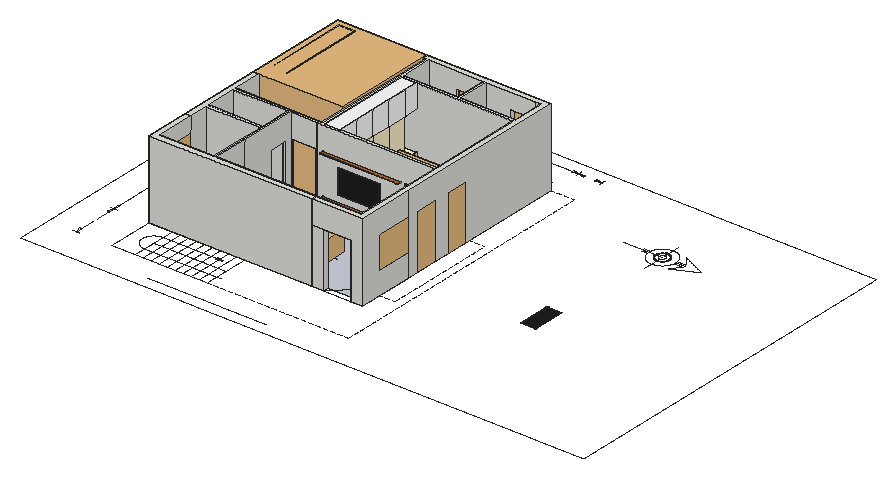
# SketchUp Ruby script. Lengths in inches.
U = 1.inch
M = Sketchup.active_model
def pt(a) = Geom::Point3d.new(a.map { |v| v * U })
def face(e, loops, mat)
  f = e.add_face(loops[0].map { |a| pt(a) })
  loops[1..].each { |l| e.add_face(l.map { |a| pt(a) }).erase! }
  f.material = f.back_material = mat if mat
  f
end
# faces: each face lists its corners as indices into pts; further lists are holes
def faces(e, pts, list, mat = nil) = list.each { |f| face(e, (f[0].is_a?(Array) ? f : [f]).map { |l| l.map { |i| pts[i] } }, mat) }
# xy, xz, yz: faces in a plane at the given z, y or x. An outline is a flat list of corners, or four numbers for a rectangle; further outlines are holes
def ring(l) = l.size == 4 ? [[l[0], l[1]], [l[2], l[1]], [l[2], l[3]], [l[0], l[3]]] : l.each_slice(2).to_a
def flat(e, list, mat, &to3) = list.each { |f| face(e, (f[0].is_a?(Array) ? f : [f]).map { |l| ring(l).map { |u, v| to3.(u, v) } }, mat) }
def xy(e, z, list, mat = nil) = flat(e, list, mat) { |x, y| [x, y, z] }
def xz(e, y, list, mat = nil) = flat(e, list, mat) { |x, z| [x, y, z] }
def yz(e, x, list, mat = nil) = flat(e, list, mat) { |y, z| [x, y, z] }
def lines(e, pts, list) = list.each { |a, b| e.add_line(pt(pts[a]), pt(pts[b])) }
# prism: a flat outline (further loops are holes) pulled along v
def prism(e, loops, v, mat = nil)
  f = face(e, loops, mat); d = Geom::Vector3d.new(v.map { |x| x * U })
  f.pushpull(f.normal.samedirection?(d) ? d.length : -d.length)
end
def box(e, o, s, mat = nil) = prism(e, [[o, [o[0] + s[0], o[1], o[2]], [o[0] + s[0], o[1] + s[1], o[2]], [o[0], o[1] + s[1], o[2]]]], [0, 0, s[2]], mat)
def at(x, y, z, deg = 0) = Geom::Transformation.translation(pt([x, y, z])) * Geom::Transformation.rotation(ORIGIN, Z_AXIS, deg.degrees)
def axes(o, x, y, z) = Geom::Transformation.new([*x, 0, *y, 0, *z, 0, *pt(o).to_a, 1])
def part(name) = M.definitions.add(name)
# library, detail: a bought-in or finely detailed component or shape, given as its bounding box
def library(name, o, s) = part(name).tap { |d| box(d.entities, o, s) }
def detail(e, o, s) = box(e.add_group.entities, o, s)
def put(e, d, t, mat = nil) = e.add_instance(d, t).tap { |i| i.material = mat if mat }
def group(e, t, mat = nil) = e.add_group.tap { |g| g.transformation = t; g.material = mat if mat }.entities
root = M.entities
M.materials.add("[Color D01]").color = [255, 242, 204]
M.materials.add("[Color L01]").color = [255, 204, 229]
M.materials.add("[Color M00]").color = [255, 255, 255]
M.materials.add("[Color M08]").color = [30, 30, 30]
M.materials.add("[Marble Carrara Floor Tile]").color = [204, 208, 219]
M.materials.add("[Marble Carrara Gold Floor Tile]").color = [225, 223, 217]
M.materials.add("[Wood Bamboo]").color = [177, 105, 43]
c1 = part("1-9-2026(1).dwg")
xy(c1.entities,0,[[43.08,54.3,41.58,63.33,44.59,63.33],[216.375,106.82,216.375,109.83,225.4,108.32],[41.58,117.35,43.08,126.24,44.59,117.35],[43.08,126.24,41.58,135.27,44.59,135.27],[630.25,455.86,632.71,456.14,635.31,455.86],
  [41.58,480.21,43.08,489.24,44.59,480.21],[106.41,540.9375,97.38,542.44,106.41,543.95],[416.88,540.9375,416.88,543.95,425.77,542.44],[434.8,540.9375,425.77,542.44,434.8,543.95],[452.85,540.9375,452.85,543.95,461.88,542.44]])
p = [[239.9,436.99,0],[239.9,281.34,0],[235.39,281.34,0],[235.39,276.83,0],[372.43,276.83,0],[372.43,281.34,0],
  [244.41,281.34,0],[244.41,427.6875,0],[378.3125,427.6875,0],[378.3125,432.2,0],[332.91,432.2,0],[332.91,480.21,0],
  [416.88,480.21,0],[416.88,432.2,0],[407.86,432.2,0],[407.86,427.6875,0],[416.88,427.6875,0],[416.88,281.34,0],
  [407.86,281.34,0],[407.86,276.83,0],[416.88,276.83,0],[416.88,267.9375,0],[425.77,267.9375,0],[425.77,489.24,0],
  [97.38,489.24,0],[97.38,126.24,0],[365.87,126.24,0],[365.87,135.27,0],[194.9,135.27,0],[194.9,159.34,0],
  [190.39,159.34,0],[190.39,135.27,0],[106.41,135.27,0],[106.41,224.44,0],[190.39,224.44,0],[190.39,189.29,0],
  [194.9,189.29,0],[194.9,237.85,0],[190.39,237.85,0],[190.39,228.96,0],[106.41,228.96,0],[106.41,276.83,0],
  [190.39,276.83,0],[190.39,267.9375,0],[194.9,267.9375,0],[194.9,276.83,0],[199.41,276.83,0],[199.41,281.34,0],
  [106.41,281.34,0],[106.41,480.21,0],[239.9,480.21,0],[239.9,466.4,0],[244.41,466.4,0],[244.41,480.21,0],
  [328.25,480.21,0],[328.25,432.2,0],[244.41,432.2,0],[244.41,436.99,0],[407.86,135.27,0],[407.86,126.24,0],
  [425.77,126.24,0],[425.77,231.83,0],[416.88,231.83,0],[416.88,135.27,0],[347.8125,135.27,0],[347.8125,126.24,0],
  [347.8125,130.75,0],[365.87,130.75,0],[97.38,54.3,0],[244.41,54.3,0],[244.41,126.24,0],[133.35,126.24,0],
  [133.35,54.3,0],[133.35,90.27,0],[244.41,90.27,0],[145.66,54.3,0],[145.66,126.24,0],[157.97,54.3,0],
  [157.97,126.24,0],[170.42,54.3,0],[170.42,126.24,0],[182.73,54.3,0],[182.73,126.24,0],[195.04,54.3,0],
  [195.04,126.24,0],[207.35,54.3,0],[207.35,126.24,0],[219.66,54.3,0],[219.66,126.24,0],[231.97,54.3,0],
  [231.97,126.24,0],[250.02,54.3,0],[253.71,54.3,0],[261.24,54.3,0],[264.93,54.3,0],[272.45,54.3,0],
  [276.28,54.3,0],[283.67,54.3,0],[287.5,54.3,0],[295.02,54.3,0],[298.71,54.3,0],[306.23,54.3,0],
  [309.93,54.3,0],[317.45,54.3,0],[321.28,54.3,0],[328.67,54.3,0],[332.49,54.3,0],[340.02,54.3,0],
  [343.71,54.3,0],[351.23,54.3,0],[354.93,54.3,0],[362.45,54.3,0],[366.28,54.3,0],[373.66,54.3,0],
  [377.49,54.3,0],[385.02,54.3,0],[388.71,54.3,0],[396.23,54.3,0],[399.92,54.3,0],[407.45,54.3,0],
  [411.28,54.3,0],[418.66,54.3,0],[422.49,54.3,0],[430.01,54.3,0],[433.71,54.3,0],[441.23,54.3,0],
  [444.92,54.3,0],[452.44,54.3,0],[456.27,54.3,0],[461.88,54.3,0],[461.88,61.82,0],[416.88,159.34,0],
  [425.77,159.34,0],[416.88,213.23,0],[425.77,213.23,0],[421.4,159.34,0],[421.4,213.23,0],[181.36,489.24,0],
  [181.36,480.21,0],[235.39,489.24,0],[235.39,480.21,0],[181.36,484.72,0],[235.39,484.72,0],[407.86,480.21,0],
  [407.86,489.24,0],[371.89,480.21,0],[371.89,489.24,0],[371.89,484.72,0],[376.67,484.72,0],[380.5,484.72,0],
  [388.02,484.72,0],[391.72,484.72,0],[399.24,484.72,0],[402.93,484.72,0],[407.86,484.72,0],[416.88,290.37,0],
  [425.77,290.37,0],[416.88,326.34,0],[425.77,326.34,0],[421.4,290.37,0],[421.4,326.34,0],[106.41,159.34,0],
  [97.38,159.34,0],[106.41,195.3125,0],[97.38,195.3125,0],[101.9,159.34,0],[101.9,195.3125,0],[97.38,290.37,0],
  [106.41,290.37,0],[97.38,326.34,0],[106.41,326.34,0],[101.9,290.37,0],[101.9,326.34,0],[163.72,364.36,0],
  [166.59,364.36,0],[318.95,348.22,0],[321.83,348.22,0],[353.15,348.22,0],[356.02,348.22,0],[327.43,197.23,0],
  [330.31,197.23,0],[241.27,489.24,0],[241.27,493.48,0],[241.27,497.31,0],[241.27,504.83,0],[241.27,508.52,0],
  [241.27,512.76,0],[232.79,512.76,0],[175.48,489.24,0],[175.48,493.48,0],[175.48,497.31,0],[175.48,504.83,0],
  [175.48,508.52,0],[175.48,512.76,0],[183.96,512.76,0],[187.79,512.76,0],[195.17,512.76,0],[199,512.76,0],
  [206.53,512.76,0],[210.22,512.76,0],[217.74,512.76,0],[221.44,512.76,0],[228.96,512.76,0],[366,489.24,0],
  [366,496.21,0],[366,499.9,0],[366,506.88,0],[371.06,506.88,0],[374.89,506.88,0],[382.28,506.88,0],
  [386.11,506.88,0],[393.63,506.88,0],[397.33,506.88,0],[404.85,506.88,0],[408.54,506.88,0],[413.74,506.88,0],
  [413.74,499.9,0],[413.74,489.24,0],[413.74,496.21,0],[425.77,332.22,0],[430.15,332.22,0],[433.84,332.22,0],
  [441.37,332.22,0],[445.2,332.22,0],[449.4375,332.22,0],[445.2,159.34,0],[449.4375,159.34,0],[449.4375,168.23,0],
  [449.4375,171.92,0],[449.4375,179.45,0],[449.4375,183.28,0],[449.4375,190.8,0],[449.4375,194.49,0],[449.4375,202.01,0],
  [449.4375,205.71,0],[449.4375,213.23,0],[449.4375,216.92,0],[449.4375,224.44,0],[449.4375,228.27,0],[449.4375,235.66,0],
  [449.4375,239.49,0],[449.4375,247.01,0],[449.4375,250.7,0],[449.4375,258.23,0],[449.4375,261.92,0],[449.4375,269.44,0],
  [449.4375,273.27,0],[449.4375,280.66,0],[449.4375,284.49,0],[449.4375,292.01,0],[449.4375,295.7,0],[449.4375,303.23,0],
  [449.4375,306.92,0],[449.4375,314.44,0],[449.4375,318.27,0],[449.4375,327.16,0],[430.15,159.34,0],[433.84,159.34,0],
  [441.37,159.34,0],[407.86,168.23,0],[405.8,126.24,0],[405.8,166.32,0],[97.38,153.32,0],[93.01,153.32,0],
  [89.3125,153.32,0],[81.79,153.32,0],[78.1,153.32,0],[73.72,153.32,0],[73.72,158.52,0],[97.38,201.19,0],
  [93.01,201.19,0],[89.3125,201.19,0],[81.79,201.19,0],[78.1,201.19,0],[73.72,201.19,0],[73.72,196,0],
  [73.72,162.35,0],[73.72,169.74,0],[73.72,173.56,0],[73.72,181.09,0],[73.72,184.78,0],[73.72,192.3,0],
  [97.38,284.49,0],[93.01,284.49,0],[89.3125,284.49,0],[81.79,284.49,0],[78.1,284.49,0],[73.72,284.49,0],
  [73.72,289.68,0],[97.38,332.22,0],[93.01,332.22,0],[89.3125,332.22,0],[81.79,332.22,0],[78.1,332.22,0],
  [73.72,332.22,0],[73.72,327.16,0],[73.72,293.38,0],[73.72,300.9,0],[73.72,304.59,0],[73.72,312.12,0],
  [73.72,315.81,0],[73.72,323.33,0],[133.43,108.33,0],[132.25,108.29,0],[131.08,108.17,0],[129.92,107.98,0],
  [128.77,107.71,0],[127.65,107.375,0],[126.54,106.96,0],[125.47,106.47,0],[124.43,105.92,0],[123.44,105.3,0],
  [122.48,104.61,0],[121.57,103.86,0],[120.71,103.06,0],[119.91,102.2,0],[119.16,101.29,0],[118.47,100.33,0],
  [117.85,99.33,0],[117.3,98.3,0],[116.8125,97.22,0],[116.4,96.125,0],[116.05,95,0],[115.79,93.85,0],
  [115.6,92.69,0],[115.48,91.52,0],[115.44,90.34,0],[115.48,89.17,0],[115.6,87.99,0],[115.79,86.83,0],
  [116.05,85.6875,0],[116.4,84.5625,0],[116.8125,83.46,0],[117.3,82.39,0],[117.85,81.35,0],[118.47,80.35,0],
  [119.16,79.39,0],[119.91,78.48,0],[120.71,77.625,0],[121.57,76.82,0],[122.48,76.07,0],[123.44,75.39,0],
  [124.43,74.77,0],[125.47,74.21,0],[126.54,73.73,0],[127.65,73.3125,0],[128.77,72.97,0],[129.92,72.7,0],
  [131.08,72.51,0],[132.25,72.39,0],[133.43,72.36,0],[216.375,108.32,0],[133.35,108.32,0],[133.35,72.35,0],
  [251.11,72.35,0],[407.86,312.25,0],[405.8,276.83,0],[405.8,310.34,0],[235.39,312.25,0],[199.96,276.83,0],
  [233.33,276.83,0],[233.33,310.34,0],[407.86,457.23,0],[405.8,427.6875,0],[405.8,455.32,0],[390.35,267.9375,0],
  [425.77,232.51,0],[425.77,265.89,0],[392.4,265.89,0],[181.09,18.6,0],[363.68,18.6,0],[269.44,436.99,0],
  [239.9,438.9,0],[267.39,438.9,0],[323.47,480.21,0],[323.47,489.24,0],[287.5,480.21,0],[287.5,489.24,0],
  [287.5,484.72,0],[292.42,484.72,0],[296.11,484.72,0],[303.64,484.72,0],[307.33,484.72,0],[314.85,484.72,0],
  [318.68,484.72,0],[323.47,484.72,0],[281.62,489.24,0],[281.62,496.21,0],[281.62,499.9,0],[281.62,506.88,0],
  [286.8125,506.88,0],[290.51,506.88,0],[298.03,506.88,0],[301.72,506.88,0],[309.24,506.88,0],[313.07,506.88,0],
  [320.46,506.88,0],[324.29,506.88,0],[329.35,506.88,0],[329.35,499.9,0],[329.35,489.24,0],[329.35,496.21,0],
  [632.71,440.27,0],[632.71,411.14,0],[642.3125,445.01,0],[642.29,445.63,0],[642.23,446.25,0],[642.13,446.86,0],
  [641.99,447.47,0],[641.81,448.0625,0],[641.59,448.65,0],[641.33,449.21,0],[641.04,449.76,0],[640.71,450.29,0],
  [640.35,450.8,0],[639.95,451.28,0],[639.53,451.73,0],[639.07,452.16,0],[638.59,452.55,0],[638.09,452.91,0],
  [637.56,453.24,0],[637.01,453.53,0],[636.44,453.79,0],[635.86,454.01,0],[635.27,454.19,0],[634.66,454.33,0],
  [634.05,454.43,0],[633.43,454.49,0],[632.81,454.51,0],[632.18,454.49,0],[631.56,454.43,0],[630.95,454.33,0],
  [630.34,454.19,0],[629.75,454.01,0],[629.17,453.79,0],[628.6,453.53,0],[628.05,453.24,0],[627.52,452.91,0],
  [627.02,452.55,0],[626.54,452.16,0],[626.08,451.73,0],[625.66,451.28,0],[625.26,450.8,0],[624.9,450.29,0],
  [624.57,449.76,0],[624.28,449.21,0],[624.02,448.65,0],[623.8,448.0625,0],[623.625,447.47,0],[623.48,446.86,0],
  [623.38,446.25,0],[623.32,445.63,0],[623.3,445.01,0],[623.32,444.39,0],[623.38,443.77,0],[623.48,443.15,0],
  [623.625,442.55,0],[623.8,441.95,0],[624.02,441.37,0],[624.28,440.8,0],[624.57,440.26,0],[624.9,439.73,0],
  [625.26,439.22,0],[625.66,438.74,0],[626.08,438.29,0],[626.54,437.86,0],[627.02,437.47,0],[627.52,437.1,0],
  [628.05,436.78,0],[628.6,436.48,0],[629.17,436.23,0],[629.75,436.01,0],[630.34,435.83,0],[630.95,435.69,0],
  [631.56,435.58,0],[632.18,435.52,0],[632.81,435.5,0],[633.43,435.52,0],[634.05,435.58,0],[634.66,435.69,0],
  [635.27,435.83,0],[635.86,436.01,0],[636.44,436.23,0],[637.01,436.48,0],[637.56,436.78,0],[638.09,437.1,0],
  [638.59,437.47,0],[639.07,437.86,0],[639.53,438.29,0],[639.95,438.74,0],[640.35,439.22,0],[640.71,439.73,0],
  [641.04,440.26,0],[641.33,440.8,0],[641.59,441.37,0],[641.81,441.95,0],[641.99,442.55,0],[642.13,443.15,0],
  [642.23,443.77,0],[642.29,444.39,0],[653.64,444.92,0],[668.82,444.92,0],[655.6875,427.14,0],[693.3,444.92,0],
  [655.6875,462.57,0],[637.39,445.01,0],[637.38,445.31,0],[637.35,445.61,0],[637.3,445.9,0],[637.23,446.19,0],
  [637.14,446.48,0],[637.04,446.76,0],[636.91,447.04,0],[636.77,447.3,0],[636.61,447.55,0],[636.44,447.8,0],
  [636.25,448.03,0],[636.05,448.25,0],[635.83,448.45,0],[635.59,448.64,0],[635.35,448.82,0],[635.1,448.98,0],
  [634.83,449.12,0],[634.56,449.24,0],[634.28,449.35,0],[633.99,449.43,0],[633.7,449.5,0],[633.4,449.55,0],
  [633.1,449.58,0],[632.81,449.59,0],[632.51,449.58,0],[632.21,449.55,0],[631.91,449.5,0],[631.62,449.43,0],
  [631.33,449.35,0],[631.05,449.24,0],[630.78,449.12,0],[630.51,448.98,0],[630.26,448.82,0],[630.02,448.64,0],
  [629.78,448.45,0],[629.57,448.25,0],[629.36,448.03,0],[629.17,447.8,0],[629,447.55,0],[628.84,447.3,0],
  [628.7,447.04,0],[628.57,446.76,0],[628.47,446.48,0],[628.38,446.19,0],[628.3125,445.9,0],[628.26,445.61,0],
  [628.23,445.31,0],[628.22,445.01,0],[628.23,444.71,0],[628.26,444.41,0],[628.3125,444.11,0],[628.38,443.82,0],
  [628.47,443.54,0],[628.57,443.26,0],[628.7,442.98,0],[628.84,442.72,0],[629,442.46,0],[629.17,442.22,0],
  [629.36,441.99,0],[629.57,441.77,0],[629.78,441.5625,0],[630.02,441.375,0],[630.26,441.2,0],[630.51,441.04,0],
  [630.78,440.9,0],[631.05,440.78,0],[631.33,440.67,0],[631.62,440.58,0],[631.91,440.51,0],[632.21,440.47,0],
  [632.51,440.4375,0],[632.81,440.43,0],[633.1,440.4375,0],[633.4,440.47,0],[633.7,440.51,0],[633.99,440.58,0],
  [634.28,440.67,0],[634.56,440.78,0],[634.83,440.9,0],[635.1,441.04,0],[635.35,441.2,0],[635.59,441.375,0],
  [635.83,441.5625,0],[636.05,441.77,0],[636.25,441.99,0],[636.44,442.22,0],[636.61,442.46,0],[636.77,442.72,0],
  [636.91,442.98,0],[637.04,443.26,0],[637.14,443.54,0],[637.23,443.82,0],[637.3,444.11,0],[637.35,444.41,0],
  [637.38,444.71,0],[653.36,448.2,0],[666.22,448.2,0],[653.36,441.5,0],[666.22,441.5,0],[632.71,449.57,0],
  [632.71,475.83,0],[644.09,445.01,0],[644.06,445.75,0],[643.99,446.48,0],[643.87,447.21,0],[643.7,447.93,0],
  [643.49,448.64,0],[643.23,449.33,0],[642.93,450,0],[642.58,450.65,0],[642.1875,451.28,0],[641.76,451.88,0],
  [641.29,452.45,0],[640.78,452.99,0],[640.25,453.49,0],[639.67,453.96,0],[639.07,454.39,0],[638.45,454.78,0],
  [637.8,455.13,0],[637.125,455.43,0],[636.43,455.69,0],[635.73,455.91,0],[635.01,456.08,0],[634.28,456.2,0],
  [633.54,456.27,0],[632.81,456.29,0],[632.07,456.27,0],[631.33,456.2,0],[630.6,456.08,0],[629.88,455.91,0],
  [629.18,455.69,0],[628.49,455.43,0],[627.81,455.13,0],[627.16,454.78,0],[626.54,454.39,0],[625.9375,453.96,0],
  [625.37,453.49,0],[624.83,452.99,0],[624.32,452.45,0],[623.85,451.88,0],[623.42,451.28,0],[623.03,450.65,0],
  [622.69,450,0],[622.38,449.33,0],[622.12,448.64,0],[621.91,447.93,0],[621.74,447.21,0],[621.62,446.48,0],
  [621.55,445.75,0],[621.52,445.01,0],[621.55,444.27,0],[621.62,443.54,0],[621.74,442.81,0],[621.91,442.09,0],
  [622.12,441.38,0],[622.38,440.69,0],[622.69,440.02,0],[623.03,439.37,0],[623.42,438.74,0],[623.85,438.14,0],
  [624.32,437.57,0],[624.83,437.03,0],[625.37,436.52,0],[625.9375,436.06,0],[626.54,435.625,0],[627.16,435.24,0],
  [627.81,434.89,0],[628.49,434.58,0],[629.18,434.32,0],[629.88,434.11,0],[630.6,433.94,0],[631.33,433.82,0],
  [632.07,433.75,0],[632.81,433.72,0],[633.54,433.75,0],[634.28,433.82,0],[635.01,433.94,0],[635.73,434.11,0],
  [636.43,434.32,0],[637.125,434.58,0],[637.8,434.89,0],[638.45,435.24,0],[639.07,435.625,0],[639.67,436.06,0],
  [640.25,436.52,0],[640.78,437.03,0],[641.29,437.57,0],[641.76,438.14,0],[642.1875,438.74,0],[642.58,439.37,0],
  [642.93,440.02,0],[643.23,440.69,0],[643.49,441.38,0],[643.7,442.09,0],[643.87,442.81,0],[643.99,443.54,0],
  [644.06,444.27,0],[626.56,435.62,0],[630.66,435.62,0],[630.25,433.98,0],[635.31,433.98,0],[607.54,444.92,0],
  [603.17,448.2,0],[612.2,448.2,0],[612.2,441.5,0],[603.17,441.5,0],[611.92,444.92,0],[632.71,444.92,0],
  [572.26,444.92,0],[653.66,445.01,0],[653.62,446.37,0],[653.48,447.73,0],[653.26,449.08,0],[652.95,450.41,0],
  [652.56,451.71,0],[652.08,452.99,0],[651.51,454.23,0],[650.87,455.4375,0],[650.15,456.6,0],[649.35,457.71,0],
  [648.49,458.76,0],[647.55,459.76,0],[646.56,460.69,0],[645.5,461.56,0],[644.39,462.35,0],[643.23,463.07,0],
  [642.03,463.72,0],[640.79,464.28,0],[639.51,464.76,0],[638.2,465.16,0],[636.875,465.47,0],[635.53,465.6875,0],
  [634.17,465.82,0],[632.81,465.87,0],[631.44,465.82,0],[630.08,465.6875,0],[628.74,465.47,0],[627.41,465.16,0],
  [626.1,464.76,0],[624.82,464.28,0],[623.58,463.72,0],[622.375,463.07,0],[621.22,462.35,0],[620.11,461.56,0],
  [619.05,460.69,0],[618.06,459.76,0],[617.125,458.76,0],[616.26,457.71,0],[615.46,456.6,0],[614.74,455.4375,0],
  [614.1,454.23,0],[613.54,452.99,0],[613.05,451.71,0],[612.66,450.41,0],[612.35,449.08,0],[612.125,447.73,0],
  [611.99,446.37,0],[611.95,445.01,0],[611.99,443.64,0],[612.125,442.29,0],[612.35,440.9375,0],[612.66,439.61,0],
  [613.05,438.3,0],[613.54,437.03,0],[614.1,435.78,0],[614.74,434.58,0],[615.46,433.42,0],[616.26,432.3125,0],
  [617.125,431.26,0],[618.06,430.26,0],[619.05,429.33,0],[620.11,428.46,0],[621.22,427.67,0],[622.375,426.95,0],
  [623.58,426.3,0],[624.82,425.74,0],[626.1,425.26,0],[627.41,424.86,0],[628.74,424.55,0],[630.08,424.33,0],
  [631.44,424.2,0],[632.81,424.15,0],[634.17,424.2,0],[635.53,424.33,0],[636.875,424.55,0],[638.2,424.86,0],
  [639.51,425.26,0],[640.79,425.74,0],[642.03,426.3,0],[643.23,426.95,0],[644.39,427.67,0],[645.5,428.46,0],
  [646.56,429.33,0],[647.55,430.26,0],[648.49,431.26,0],[649.35,432.3125,0],[650.15,433.42,0],[650.87,434.58,0],
  [651.51,435.78,0],[652.08,437.03,0],[652.56,438.3,0],[652.95,439.61,0],[653.26,440.9375,0],[653.48,442.29,0],
  [653.62,443.64,0],[0,563.23,0],[867.82,563.23,0],[867.82,0,0],[0,0,0],[430.7,489.24,0],
  [434.53,489.24,0],[441.91,489.24,0],[445.74,489.24,0],[453.27,489.24,0],[456.96,489.24,0],[461.88,489.24,0],
  [461.88,481.71,0],[461.88,478.02,0],[461.88,470.5,0],[461.88,466.67,0],[461.88,459.15,0],[461.88,455.45,0],
  [461.88,447.93,0],[461.88,444.24,0],[461.88,436.72,0],[461.88,433.02,0],[461.88,425.5,0],[461.88,421.67,0],
  [461.88,414.28,0],[461.88,410.46,0],[461.88,402.93,0],[461.88,399.24,0],[461.88,391.72,0],[461.88,388.02,0],
  [461.88,380.5,0],[461.88,376.67,0],[461.88,369.29,0],[461.88,365.46,0],[461.88,357.93,0],[461.88,354.24,0],
  [461.88,346.72,0],[461.88,343.03,0],[461.88,335.5,0],[461.88,331.8125,0],[461.88,324.29,0],[461.88,320.46,0],
  [461.88,312.9375,0],[461.88,309.24,0],[461.88,301.72,0],[461.88,298.03,0],[461.88,290.51,0],[461.88,286.8125,0],
  [461.88,279.29,0],[461.88,275.46,0],[461.88,268.07,0],[461.88,264.25,0],[461.88,256.72,0],[461.88,253.03,0],
  [461.88,245.51,0],[461.88,241.8125,0],[461.88,234.29,0],[461.88,230.46,0],[461.88,223.08,0],[461.88,219.25,0],
  [461.88,211.72,0],[461.88,208.03,0],[461.88,200.51,0],[461.88,196.82,0],[461.88,189.29,0],[461.88,185.46,0],
  [461.88,178.08,0],[461.88,174.25,0],[461.88,166.73,0],[461.88,163.03,0],[461.88,155.51,0],[461.88,151.82,0],
  [461.88,144.3,0],[461.88,140.6,0],[461.88,133.08,0],[461.88,129.25,0],[461.88,121.73,0],[461.88,118.03,0],
  [461.88,110.51,0],[461.88,106.82,0],[461.88,99.3,0],[461.88,95.6,0],[461.88,88.08,0],[461.88,84.25,0],
  [461.88,76.87,0],[461.88,73.04,0],[461.88,65.51,0],[97.38,537.38,0],[97.38,548.46,0],[425.77,548.46,0],
  [425.77,537.38,0],[106.41,542.44,0],[248.65,542.44,0],[416.88,542.44,0],[274.5,542.44,0],[267.25,542.44,0],
  [271.36,542.44,0],[461.88,537.38,0],[461.88,548.46,0],[434.8,542.44,0],[435.62,542.44,0],[452.85,542.44,0],
  [452.03,542.44,0],[37.07,126.24,0],[48.01,126.24,0],[48.01,489.24,0],[37.07,489.24,0],[43.08,135.27,0],
  [43.08,303.91,0],[43.08,480.21,0],[43.08,311.71,0],[48.01,54.3,0],[37.07,54.3,0],[43.08,117.35,0],
  [43.08,94.24,0],[43.08,63.33,0],[43.08,86.44,0]]
lines(c1.entities,p,[[0,1],[1,2],[2,3],[3,4],[4,5],[5,6],[6,7],[7,8],[8,9],[9,10],[10,11],[11,12],
  [12,13],[13,14],[14,15],[15,16],[16,17],[17,18],[18,19],[19,20],[20,21],[21,22],[22,23],[23,24],
  [24,25],[25,26],[26,27],[27,28],[28,29],[29,30],[30,31],[31,32],[32,33],[33,34],[34,35],[35,36],
  [36,37],[37,38],[38,39],[39,40],[40,41],[41,42],[42,43],[43,44],[44,45],[45,46],[46,47],[47,48],
  [48,49],[49,50],[50,51],[51,52],[52,53],[53,54],[54,55],[55,56],[56,57],[57,0],[58,59],[59,60],
  [60,61],[61,62],[62,63],[63,58],[64,65],[66,67],[25,68],[68,69],[69,70],[71,72],[73,74],[75,76],
  [77,78],[79,80],[81,82],[83,84],[85,86],[87,88],[89,90],[69,91],[92,93],[94,95],[96,97],[98,99],
  [100,101],[102,103],[104,105],[106,107],[108,109],[110,111],[112,113],[114,115],[116,117],[118,119],[120,121],[122,123],
  [124,125],[126,127],[128,129],[129,130],[131,132],[133,134],[135,136],[137,138],[139,140],[141,142],[143,144],[145,146],
  [147,148],[149,150],[151,152],[153,154],[155,156],[157,158],[159,160],[161,162],[163,164],[165,166],[167,168],[169,170],
  [171,172],[173,174],[175,176],[177,178],[179,180],[181,182],[183,184],[185,186],[186,187],[188,189],[190,191],[192,193],
  [193,194],[195,196],[197,198],[199,200],[201,202],[203,204],[205,206],[206,207],[208,209],[210,211],[212,213],[214,215],
  [215,216],[217,218],[219,220],[221,222],[223,224],[225,226],[226,227],[228,229],[230,231],[232,233],[234,235],[236,237],
  [238,239],[240,241],[242,243],[244,245],[246,247],[248,249],[250,251],[252,253],[254,255],[132,256],[257,258],[26,59],
  [59,259],[259,26],[260,261],[262,263],[264,265],[266,267],[267,268],[269,270],[271,272],[273,274],[274,275],[276,277],
  [278,279],[280,281],[282,283],[284,285],[286,287],[287,288],[289,290],[291,292],[293,294],[294,295],[296,297],[298,299],
  [300,301],[302,303],[303,304],[304,305],[305,306],[306,307],[307,308],[308,309],[309,310],[310,311],[311,312],[312,313],
  [313,314],[314,315],[315,316],[316,317],[317,318],[318,319],[319,320],[320,321],[321,322],[322,323],[323,324],[324,325],
  [325,326],[326,327],[327,328],[328,329],[329,330],[330,331],[331,332],[332,333],[333,334],[334,335],[335,336],[336,337],
  [337,338],[338,339],[339,340],[340,341],[341,342],[342,343],[343,344],[344,345],[345,346],[346,347],[347,348],[348,349],
  [349,350],[351,352],[353,354],[19,355],[355,4],[356,357],[3,358],[358,359],[360,361],[15,362],[362,8],[8,15],
  [363,364],[61,22],[22,365],[365,366],[367,368],[369,370],[0,371],[371,51],[51,0],[372,373],[374,375],[376,377],
  [378,379],[380,381],[382,383],[384,385],[386,387],[388,389],[389,390],[391,392],[393,394],[395,396],[397,398],[398,399],
  [400,401],[402,403],[404,405],[405,406],[406,407],[407,408],[408,409],[409,410],[410,411],[411,412],[412,413],[413,414],
  [414,415],[415,416],[416,417],[417,418],[418,419],[419,420],[420,421],[421,422],[422,423],[423,424],[424,425],[425,426],
  [426,427],[427,428],[428,429],[429,430],[430,431],[431,432],[432,433],[433,434],[434,435],[435,436],[436,437],[437,438],
  [438,439],[439,440],[440,441],[441,442],[442,443],[443,444],[444,445],[445,446],[446,447],[447,448],[448,449],[449,450],
  [450,451],[451,452],[452,453],[453,454],[454,455],[455,456],[456,457],[457,458],[458,459],[459,460],[460,461],[461,462],
  [462,463],[463,464],[464,465],[465,466],[466,467],[467,468],[468,469],[469,470],[470,471],[471,472],[472,473],[473,474],
  [474,475],[475,476],[476,477],[477,478],[478,479],[479,480],[480,481],[481,482],[482,483],[483,484],[484,485],[485,486],
  [486,487],[487,488],[488,489],[489,490],[490,491],[491,492],[492,493],[493,494],[494,495],[495,496],[496,497],[497,498],
  [498,499],[499,404],[500,501],[501,502],[502,503],[503,504],[504,501],[505,506],[506,507],[507,508],[508,509],[509,510],
  [510,511],[511,512],[512,513],[513,514],[514,515],[515,516],[516,517],[517,518],[518,519],[519,520],[520,521],[521,522],
  [522,523],[523,524],[524,525],[525,526],[526,527],[527,528],[528,529],[529,530],[530,531],[531,532],[532,533],[533,534],
  [534,535],[535,536],[536,537],[537,538],[538,539],[539,540],[540,541],[541,542],[542,543],[543,544],[544,545],[545,546],
  [546,547],[547,548],[548,549],[549,550],[550,551],[551,552],[552,553],[553,554],[554,555],[555,556],[556,557],[557,558],
  [558,559],[559,560],[560,561],[561,562],[562,563],[563,564],[564,565],[565,566],[566,567],[567,568],[568,569],[569,570],
  [570,571],[571,572],[572,573],[573,574],[574,575],[575,576],[576,577],[577,578],[578,579],[579,580],[580,581],[581,582],
  [582,583],[583,584],[584,585],[585,586],[586,587],[587,588],[588,589],[589,590],[590,591],[591,592],[592,593],[593,594],
  [594,595],[595,596],[596,597],[597,598],[598,599],[599,600],[600,505],[601,602],[603,604],[605,606],[607,608],[608,609],
  [609,610],[610,611],[611,612],[612,613],[613,614],[614,615],[615,616],[616,617],[617,618],[618,619],[619,620],[620,621],
  [621,622],[622,623],[623,624],[624,625],[625,626],[626,627],[627,628],[628,629],[629,630],[630,631],[631,632],[632,633],
  [633,634],[634,635],[635,636],[636,637],[637,638],[638,639],[639,640],[640,641],[641,642],[642,643],[643,644],[644,645],
  [645,646],[646,647],[647,648],[648,649],[649,650],[650,651],[651,652],[652,653],[653,654],[654,655],[655,656],[656,657],
  [657,658],[658,659],[659,660],[660,661],[661,662],[662,663],[663,664],[664,665],[665,666],[666,667],[667,668],[668,669],
  [669,670],[670,671],[671,672],[672,673],[673,674],[674,675],[675,676],[676,677],[677,678],[678,679],[679,680],[680,681],
  [681,682],[682,683],[683,684],[684,685],[685,686],[686,687],[687,688],[688,689],[689,690],[690,691],[691,692],[692,693],
  [693,694],[694,695],[695,696],[696,697],[697,698],[698,699],[699,700],[700,701],[701,702],[702,607],[703,704],[705,706],
  [707,708],[708,709],[710,711],[711,707],[707,712],[713,714],[715,716],[716,717],[717,718],[718,719],[719,720],[720,721],
  [721,722],[722,723],[723,724],[724,725],[725,726],[726,727],[727,728],[728,729],[729,730],[730,731],[731,732],[732,733],
  [733,734],[734,735],[735,736],[736,737],[737,738],[738,739],[739,740],[740,741],[741,742],[742,743],[743,744],[744,745],
  [745,746],[746,747],[747,748],[748,749],[749,750],[750,751],[751,752],[752,753],[753,754],[754,755],[755,756],[756,757],
  [757,758],[758,759],[759,760],[760,761],[761,762],[762,763],[763,764],[764,765],[765,766],[766,767],[767,768],[768,769],
  [769,770],[770,771],[771,772],[772,773],[773,774],[774,775],[775,776],[776,777],[777,778],[778,779],[779,780],[780,781],
  [781,782],[782,783],[783,784],[784,785],[785,786],[786,787],[787,788],[788,789],[789,790],[790,791],[791,792],[792,793],
  [793,794],[794,795],[795,796],[796,797],[797,798],[798,799],[799,800],[800,801],[801,802],[802,803],[803,804],[804,805],
  [805,806],[806,807],[807,808],[808,809],[809,810],[810,715],[811,812],[812,813],[813,814],[814,811],[23,815],[816,817],
  [818,819],[820,821],[821,822],[823,824],[825,826],[827,828],[829,830],[831,832],[833,834],[835,836],[837,838],[839,840],
  [841,842],[843,844],[845,846],[847,848],[849,850],[851,852],[853,854],[855,856],[857,858],[859,860],[861,862],[863,864],
  [865,866],[867,868],[869,870],[871,872],[873,874],[875,876],[877,878],[879,880],[881,882],[883,884],[885,886],[887,888],
  [889,890],[891,892],[893,894],[895,896],[897,898],[899,900],[901,902],[903,904],[905,906],[907,908],[909,910],[911,912],
  [913,914],[915,916],[917,918],[919,920],[921,922],[923,924],[925,926]])
c2 = library("Bed 003",[-38.05,-87.1,0],[75.86,87.1,55.12])
c3 = library("Sofa 142 022",[-42.35,-14.43,0],[84.7,28.86,43.89])
c4 = library("Table 83-05",[-30.14,-14.6875,0],[60.28,29.375,31.83])
c5 = library("Kitchen Cabinets Island 86-03",[-53.9375,-10.44,0],[107.875,20.88,31.52])
c6 = library("Window 46-10",[-43.56,-2.12,0],[87.13,4.27,82.67])
c7 = library("Door 243 067",[-20.85,-3,0],[41.7,6,82.46])
c8 = library("Group\#3",[0,0,0],[138,162.9,120.25])
c9 = part("Group\#14")
box(c9.entities,[0,0.2,0],[0.71,30.39,11.8],"[Color M00]")
c10 = part("Group\#21")
box(c10.entities,[0,0.2,0],[0.71,30.39,11.8],"[Color M00]")
c11 = part("Group\#15")
box(c11.entities,[0,-0.07,0],[0.71,30.66,36.25],"[Color M00]")
xy(root,0,[[306.23,71.94,324.29,80.97],[366.28,71.94,384.19,80.97],[375.3,80.97,384.19,158.93],[375.3,158.93,384.19,177.53],[375.3,213.64,384.19,236.07],
  [193.81,222.53,193.81,227.04,198.32,227.04,198.32,382.69,202.83,382.69,202.83,222.53],[202.83,222.53,330.85,227.04],[366.28,222.53,375.3,227.04],[55.8,236.07,64.83,272.04],[375.3,236.07,384.19,272.04],
  [375.3,272.04,375.3,373.39,366.28,373.39,366.28,377.9,375.3,377.9,375.3,425.91,366.28,425.91,366.28,434.9375,384.19,434.9375,384.19,272.04],[202.83,373.39,202.83,377.9,286.68,377.9,286.68,425.91,291.33,425.91,291.33,377.9,336.73,377.9,336.73,373.39],[198.32,412.1,202.83,425.91],[139.78,425.91,193.81,434.9375],[193.81,425.91,281.89,434.9375]])
xy(root,0,[[64.83,80.97,148.81,80.97,148.81,105.04,153.32,105.04,153.32,80.97,375.3,80.97,375.3,177.53,384.19,177.53,384.19,213.64,375.3,213.64,375.3,222.53,366.28,222.53,366.28,227.04,375.3,227.04,375.3,373.39,202.83,373.39,202.83,227.04,330.85,227.04,330.85,222.53,64.83,222.53,64.83,174.66,148.81,174.66,148.81,183.55,153.32,183.55,153.32,134.99,148.81,134.99,148.81,170.15,64.83,170.15],[336.73,373.39,366.28,373.39,366.28,377.9,375.3,377.9,375.3,425.91,291.33,425.91,291.33,377.9,336.73,377.9],[202.83,377.9,286.68,425.91]],"[Marble Carrara Floor Tile]")
xy(root,0,[[64.83,222.53,193.81,222.53,193.81,227.04,198.32,227.04,198.32,382.69,202.83,382.69,202.83,412.1,198.32,412.1,198.32,425.91,88.83,425.91,88.83,296.04,64.83,296.04],[64.83,296.04,88.83,425.91]],"[Marble Carrara Gold Floor Tile]")
xy(root,36,[[375.3,105.04,384.19,158.93]])
xy(root,72.25,[[245.92,425.91,281.89,434.9375],[330.31,425.91,366.28,434.9375]])
xy(root,83.25,[[202.83,216.53,323.43,222.53]],"[Wood Bamboo]")
xy(root,83.875,[[375.3,105.04,384.19,158.93]])
xy(root,84.25,[[375.3,177.53,384.19,213.64],[330.85,222.53,366.28,227.04],[375.3,236.07,384.19,272.04],[336.73,373.39,366.28,377.9],[198.32,382.69,202.83,412.1]])
xy(root,84.25,[[202.83,216.53,323.43,222.53]],"[Wood Bamboo]")
xy(root,84.61,[[324.29,71.94,366.28,80.97]])
xy(root,96.25,[[245.92,425.91,281.89,434.9375],[330.31,425.91,366.28,434.9375]])
xy(root,120.25,[[[306.23,71.94,384.19,71.94,384.19,434.9375,366.28,434.9375,366.28,425.91,375.3,425.91,375.3,377.9,291.33,377.9,291.33,425.91,286.68,425.91,286.68,377.9,202.83,377.9,202.83,425.91,366.28,425.91,366.28,434.9375,193.81,434.9375,193.81,425.91,198.32,425.91,198.32,227.04,193.81,227.04,193.81,222.53,375.3,222.53,375.3,80.97,306.23,80.97],[202.83,227.04,375.3,373.39]]])
xz(root,71.94,[[306.23,0,324.29,84.61],[366.28,0,384.19,0,384.19,120.25,306.23,120.25,306.23,84.61,366.28,84.61]])
xz(root,80.97,[[306.23,0,324.29,84.61],[366.28,0,366.28,84.61,306.23,84.61,306.23,120.25,375.3,120.25,375.3,0]])
xz(root,105.04,[[375.3,36,384.19,83.875]])
xz(root,158.93,[[375.3,36,384.19,83.875]])
xz(root,177.53,[[375.3,0,384.19,84.25]])
xz(root,213.64,[[375.3,0,384.19,84.25]])
xz(root,216.53,[[202.83,83.25,323.43,84.25]],"[Wood Bamboo]")
xz(root,222.53,[[[193.81,0,330.85,0,330.85,84.25,366.28,84.25,366.28,0,375.3,0,375.3,120.25,193.81,120.25],[202.83,83.25,323.43,84.25]]])
xz(root,227.04,[[193.81,0,198.32,120.25],[202.83,0,202.83,120.25,375.3,120.25,375.3,0,366.28,0,366.28,84.25,330.85,84.25,330.85,0]])
xz(root,236.07,[[375.3,0,384.19,84.25]])
xz(root,272.04,[[375.3,0,384.19,84.25]])
xz(root,373.39,[[202.83,0,336.73,0,336.73,84.25,366.28,84.25,366.28,0,375.3,0,375.3,120.25,202.83,120.25]])
xz(root,377.9,[[202.83,0,286.68,120.25],[291.33,0,291.33,120.25,375.3,120.25,375.3,0,366.28,0,366.28,84.25,336.73,84.25,336.73,0]])
xz(root,382.69,[[198.32,0,202.83,84.25]])
xz(root,412.1,[[198.32,0,202.83,84.25]])
xz(root,425.91,[[193.81,0,198.32,120.25],[[202.83,0,286.68,120.25],[245.92,72.25,281.89,96.25]],[286.68,0,291.33,120.25],[291.33,0,366.28,0,366.28,72.25,330.31,72.25,330.31,96.25,366.28,96.25,366.28,120.25,291.33,120.25],[366.28,0,375.3,120.25]])
xz(root,434.9375,[[[193.81,0,193.81,120.25,366.28,120.25,366.28,96.25,330.31,96.25,330.31,72.25,366.28,72.25,366.28,0],[245.92,72.25,281.89,96.25]],[366.28,0,384.19,120.25]])
yz(root,193.81,[[222.53,0,227.04,120.25],[425.91,0,434.9375,120.25]])
yz(root,198.32,[[227.04,0,227.04,120.25,425.91,120.25,425.91,0,412.1,0,412.1,84.25,382.69,84.25,382.69,0]])
yz(root,202.83,[[227.04,0,373.39,120.25],[377.9,0,382.69,0,382.69,84.25,412.1,84.25,412.1,0,425.91,0,425.91,120.25,377.9,120.25],[216.53,83.25,222.53,84.25]])
yz(root,245.92,[[425.91,72.25,434.9375,96.25]])
yz(root,281.89,[[425.91,72.25,434.9375,96.25]])
yz(root,286.68,[[377.9,0,425.91,120.25]])
yz(root,291.33,[[377.9,0,425.91,120.25]])
yz(root,306.23,[[71.94,0,80.97,84.61],[71.94,84.61,80.97,120.25]])
yz(root,323.43,[[216.53,83.25,222.53,84.25]])
yz(root,324.29,[[71.94,0,80.97,84.61]])
yz(root,330.31,[[425.91,72.25,434.9375,96.25]])
yz(root,330.85,[[222.53,0,227.04,84.25]])
yz(root,336.73,[[373.39,0,377.9,84.25]])
yz(root,366.28,[[71.94,0,80.97,84.61],[222.53,0,227.04,84.25],[373.39,0,377.9,84.25],[425.91,72.25,434.9375,96.25]])
yz(root,375.3,[[[80.97,0,80.97,120.25,222.53,120.25,222.53,0,213.64,0,213.64,84.25,177.53,84.25,177.53,0],[105.04,36,158.93,83.875]],[227.04,0,227.04,120.25,373.39,120.25,373.39,0,272.04,0,272.04,84.25,236.07,84.25,236.07,0],[377.9,0,425.91,120.25]])
yz(root,384.19,[[71.94,0,158.93,0,158.93,36,105.04,36,105.04,83.875,158.93,83.875,158.93,120.25,71.94,120.25],[158.93,0,177.53,0,177.53,84.25,213.64,84.25,213.64,0,236.07,0,236.07,84.25,272.04,84.25,272.04,0,434.9375,0,434.9375,120.25,158.93,120.25]])
p = [[202.83,373.39,84],[202.125,349.39,84],[202.125,349.39,24.875],[202.83,373.39,24.875],[202.83,349.39,0],[202.125,349.39,0],
  [88.83,227.04,0],[64.83,227.04,0]]
faces(root,p,[[0,1,2,3]])
lines(root,p,[[4,5],[6,7]])
put(root,c1,at(-41.58,-54.3,0))
put(root,c2,at(131.25,273.1,0,-180))
put(root,c2,at(278.84,235.99,0,-180))
put(root,c3,at(249.09,106.2,0,-180))
put(root,c4,at(254.23,146.96,0,-180))
put(root,c5,axes([75.27,125.56,0],[0,0.82667,0],[-1,0,0],[0,0,1]))
put(root,c6,axes([166.8,432.82,36],[-0.62005,0,0],[0,-1,0],[0,0,0.58062]))
put(root,c6,axes([382.08,131.91,36],[0,0.62005,0],[-1,0,0],[0,0,0.58062]))
put(root,c6,axes([62.71,254.05,36],[0,0.41284,0],[-1,0,0],[0,0,0.58062]))
put(root,c6,axes([61.86,122.76,72.78],[0,0.41284,0],[-1,0,0],[0,0,0.28396]))
put(root,c6,axes([263.91,432.82,72.25],[-0.41284,0,0],[0,-1,0],[0,0,0.28396]))
put(root,c6,axes([348.29,432.82,72.25],[-0.41284,0,0],[0,-1,0],[0,0,0.28396]))
put(root,c7,axes([348.57,224.04,0],[-0.84956,0,0],[0,-1,0],[0,0,1.02166]))
put(root,c7,axes([175.55,224.04,0],[-0.84956,0,0],[0,-1,0],[0,0,1.02166]))
put(root,c7,axes([351.4,376.01,-0.07],[-0.7135,0,0],[0,-1,0],[0,0,1.02166]))
put(root,c7,axes([381.19,254.06,0],[0,0.86268,0],[-1,0,0],[0,0,1.02166]))
put(root,c7,axes([381.19,195.59,0],[0,0.86596,0],[-1,0,0],[0,0,1.02166]))
put(root,c7,axes([199.83,397.39,0],[0,0.70523,0],[-1,0,0],[0,0,1.02166]))
g1 = group(root,at(55.8,71.94,0))
xy(g1,0,[[0,0,0,69.07,9.03,69.07,9.03,9.03,93.01,9.03,93.01,33.1,97.52,33.1,97.52,9.03,250.43,9.03,250.43,0]])
xy(g1,72.25,[[0,33.1,9.03,69.07]])
xy(g1,84.25,[[93.01,33.1,97.52,63.05]])
xy(g1,96.25,[[0,33.1,9.03,69.07]])
xy(g1,120.25,[[0,0,250.43,0,250.43,9.03,97.52,9.03,97.52,63.05,93.01,63.05,93.01,9.03,9.03,9.03,9.03,69.07,0,69.07]])
xz(g1,0,[[0,0,250.43,120.25]])
xz(g1,9.03,[[9.03,0,93.01,120.25],[97.52,0,250.43,120.25]])
xz(g1,33.1,[[93.01,0,97.52,84.25],[0,72.25,9.03,96.25]])
xz(g1,63.05,[[93.01,84.25,97.52,120.25]])
xz(g1,69.07,[[0,0,9.03,72.25],[0,96.25,9.03,120.25]])
yz(g1,0,[[0,0,0,120.25,69.07,120.25,69.07,96.25,33.1,96.25,33.1,72.25,69.07,72.25,69.07,0]])
yz(g1,9.03,[[9.03,0,69.07,0,69.07,72.25,33.1,72.25,33.1,96.25,69.07,96.25,69.07,120.25,9.03,120.25]])
yz(g1,93.01,[[9.03,0,9.03,120.25,63.05,120.25,63.05,84.25,33.1,84.25,33.1,0]])
yz(g1,97.52,[[9.03,0,33.1,0,33.1,84.25,63.05,84.25,63.05,120.25,9.03,120.25]])
yz(g1,250.43,[[0,0,9.03,120.25]])
g2 = group(root,at(55.8,134.99,0))
xy(g2,0,[[93.01,0,93.01,35.15,9.03,35.15,9.03,6.02,0,6.02,0,137.05,9.03,137.05,9.03,92.05,102.03,92.05,102.03,87.53,97.52,87.53,97.52,78.64,93.01,78.64,93.01,87.53,9.03,87.53,9.03,39.66,93.01,39.66,93.01,48.55,97.52,48.55,97.52,0]])
xy(g2,36,[[0,101.08,9.03,137.05]])
xy(g2,84,[[0,101.08,9.03,137.05]])
xy(g2,84.25,[[93.01,48.55,97.52,78.64],[102.03,87.53,138,92.05]])
xy(g2,120.25,[[[93.01,0,97.52,0,97.52,87.53,138,87.53,138,92.05,9.03,92.05,9.03,137.05,0,137.05,0,6.02,9.03,6.02,9.03,35.15,93.01,35.15],[9.03,39.66,93.01,87.53]]])
xz(g2,0,[[93.01,0,97.52,120.25]])
xz(g2,6.02,[[0,0,9.03,120.25]])
xz(g2,35.15,[[9.03,0,93.01,120.25]])
xz(g2,39.66,[[9.03,0,93.01,120.25]])
xz(g2,48.55,[[93.01,0,97.52,84.25]])
xz(g2,78.64,[[93.01,0,97.52,84.25]])
xz(g2,87.53,[[9.03,0,93.01,120.25],[97.52,0,102.03,0,102.03,84.25,138,84.25,138,120.25,97.52,120.25]])
xz(g2,92.05,[[9.03,0,9.03,120.25,138,120.25,138,84.25,102.03,84.25,102.03,0]])
xz(g2,101.08,[[0,36,9.03,84]])
xz(g2,137.05,[[0,0,9.03,36],[0,84,9.03,120.25]])
yz(g2,0,[[6.02,0,6.02,120.25,137.05,120.25,137.05,84,101.08,84,101.08,36,137.05,36,137.05,0]])
yz(g2,9.03,[[6.02,0,35.15,120.25],[39.66,0,87.53,120.25],[92.05,0,137.05,0,137.05,36,101.08,36,101.08,84,137.05,84,137.05,120.25,92.05,120.25]])
yz(g2,93.01,[[0,0,35.15,120.25],[39.66,0,39.66,120.25,87.53,120.25,87.53,0,78.64,0,78.64,84.25,48.55,84.25,48.55,0]])
yz(g2,97.52,[[0,0,48.55,0,48.55,84.25,78.64,84.25,78.64,0,87.53,0,87.53,120.25,0,120.25]])
yz(g2,102.03,[[87.53,0,92.05,84.25]])
yz(g2,138,[[87.53,84.25,92.05,120.25]])
put(root,c8,at(55.8,272.04,0))
g3 = group(root,at(323.43,222.53,9,180),"[Wood Bamboo]")
prism(g3,[[[96.45,11.29,0],[120.6,11.29,0],[120.6,0,0],[0,0,0],[0,11.29,0],[24.15,11.29,0],[48.3,11.29,0],[72.3,11.29,0]]],[0,0,12],"[Color M00]")
g4 = group(g3,at(72.45,11.29,0))
box(g4,[0,0,0],[23.99,0.71,12],"[Wood Bamboo]")
g5 = group(g3,at(48.3,11.29,0))
box(g5,[0,0,0],[23.99,0.71,12],"[Wood Bamboo]")
g6 = group(g3,at(0,0,12))
xy(g6,0,[[0,0,120.6,12]],"[Color M00]")
xy(g6,1,[[0,0,120.6,12]],"[Wood Bamboo]")
xz(g6,0,[[0,0,120.6,1]],"[Color M00]")
xz(g6,12,[[0,0,120.6,1]],"[Wood Bamboo]")
yz(g6,0,[[0,0,12,1]],"[Color M00]")
yz(g6,120.6,[[0,0,12,1]],"[Color M00]")
g7 = group(g3,at(24.15,11.29,0))
xy(g7,0,[[0,0,23.99,0.71]],"[Color M00]")
xy(g7,12,[[0,0,23.99,0.71]],"[Color M00]")
xz(g7,0,[[0,0,23.99,12]],"[Color M00]")
xz(g7,0.71,[[0,0,23.99,12]],"[Wood Bamboo]")
yz(g7,0,[[0,0,0.71,12]],"[Color M00]")
yz(g7,23.99,[[0,0,0.71,12]],"[Color M00]")
g8 = group(g3,at(0,11.29,0))
xy(g8,0,[[0,0,23.99,0.71]],"[Color M00]")
xy(g8,12,[[0,0,23.99,0.71]],"[Color M00]")
xz(g8,0,[[0,0,23.99,12]],"[Color M00]")
xz(g8,0.71,[[0,0,23.99,12]],"[Wood Bamboo]")
yz(g8,0,[[0,0,0.71,12]],"[Color M00]")
yz(g8,23.99,[[0,0,0.71,12]],"[Color M00]")
g9 = group(g3,at(96.61,11.29,0))
box(g9,[0,0,0],[23.99,0.71,12],"[Wood Bamboo]")
g10 = group(root,at(88.83,425.91,0,180))
xy(g10,0,[[2.4375,0,24,129.87]],"[Color L01]")
xy(g10,4,[[0,0,2.4375,129.87]],"[Color L01]")
xy(g10,4.71,[[0,0.71,1.5,129.16],[1.5,0.71,3,97.05],[3,0.71,23.29,129.16],[1.5,97.05,3,129.16]],"[Color L01]")
xy(g10,83.29,[[0,0.71,23.29,129.16]],"[Color L01]")
xy(g10,84,[[0,0,24,129.87]],"[Color L01]")
xz(g10,0,[[2.4375,0,24,0,24,84,0,84,0,4,2.4375,4]],"[Color L01]")
xz(g10,0.71,[[0,4.71,23.29,83.29]],"[Color L01]")
xz(g10,129.16,[[0,4.71,23.29,83.29]],"[Color L01]")
xz(g10,129.87,[[2.4375,0,2.4375,4,0,4,0,84,24,84,24,0]],"[Color L01]")
yz(g10,0,[[[0,4,129.87,84],[0.71,4.71,129.16,83.29]]],"[Color L01]")
yz(g10,2.4375,[[0,0,129.87,4]],"[Color L01]")
yz(g10,23.29,[[0.71,4.71,129.16,83.29]],"[Color L01]")
yz(g10,24,[[0,0,129.87,84]],"[Color L01]")
g11 = group(g10,at(0,32.82,4.71))
box(g11,[0,0,0],[1.5,32.11,78.58],"[Color L01]")
g12 = group(g10,at(1.5,0.71,4.71))
box(g12,[0,0,0],[1.5,32.11,78.58],"[Color L01]")
g13 = group(g10,at(0,97.05,4.71),"[Color L01]")
box(g13,[0,0,0],[1.5,32.11,78.58],"[Color L01]")
g14 = group(g10,at(1.5,64.93,4.71),"[Color L01]")
box(g14,[0,0,0],[1.5,32.11,78.58],"[Color L01]")
g15 = group(root,at(89.54,425.91,84,180),"[Color L01]")
xy(g15,0,[[0.71,0,24.71,129.87]],"[Color L01]")
xy(g15,36,[[0.71,0,24.71,129.87]],"[Color L01]")
xz(g15,0,[[0.71,0,24.71,36]],"[Color L01]")
xz(g15,129.87,[[0.71,0,24.71,36]],"[Color L01]")
yz(g15,0.71,[[0,0,43.29,36],[43.29,0,129.87,36]],"[Color L01]")
yz(g15,24.71,[[0,0,129.87,36]],"[Color L01]")
g16 = group(g15,at(0,28.91,0))
xy(g16,0,[[0,0,0.71,43.13]],"[Color M00]")
xy(g16,36,[[0,0,0.71,43.13]],"[Color M00]")
xz(g16,0,[[0,0,0.71,36]],"[Color M00]")
xz(g16,43.13,[[0,0,0.71,36]],"[Color M00]")
yz(g16,0,[[0,0,43.13,36]],"[Color L01]")
yz(g16,0.71,[[0,0,43.13,36]],"[Color M00]")
g17 = group(g15,at(0,86.74,0),"[Color L01]")
box(g17,[0,0,0],[0.71,43.13,36],"[Color L01]")
g18 = group(g15,at(0,57.82,0))
box(g18,[0,0,0],[0.71,43.13,36],"[Color L01]")
g19 = group(g15,at(0,0,0))
box(g19,[0,0,0],[0.71,43.13,36],"[Color L01]")
g20 = group(root,at(226.83,373.39,84.25))
prism(g20,[[[-0.6875,-146.35,0],[-24,-146.35,0],[-24,0,0],[-0.6875,0,0],[-0.6875,-29.27,0],[-0.6875,-58.54,0],[-0.6875,-87.81,0],[-0.6875,-117.08,0]]],[0,0,36],"[Color M00]")
g21 = group(root,at(226.83,349.39,0,180),"[Color L01]")
xy(g21,0,[[0.71,0,24.71,122.35]],"[Color L01]")
xy(g21,84,[[0.71,0,24.71,122.35]],"[Color L01]")
xz(g21,0,[[0.71,0,24.71,84],[0.15,4,0.71,16],[0.15,16,0.71,28],[0.15,28,0.71,84]],"[Color L01]")
xz(g21,122.35,[[0.71,0,24.71,84]],"[Color L01]")
yz(g21,0.71,[[0,0,122.35,4],[0,4,30.59,16],[30.59,4,61.17,16],[61.17,4,91.76,16],[91.76,4,122.35,16],
  [0,16,30.59,28],[30.59,16,61.17,28],[61.17,16,91.76,28],[91.76,16,122.35,28],[0,28,30.59,84],
  [30.59,28,61.17,84],[61.17,28,91.76,84],[91.76,28,122.35,84]],"[Color L01]")
yz(g21,24.71,[[0,0,122.35,84]],"[Color L01]")
g22 = group(g21,at(0,30.46,28))
box(g22,[0,0.2,0],[0.71,30.39,56],"[Color D01]")
g23 = group(g21,at(0,91.76,28),"[Color D01]")
box(g23,[0,0.2,0],[0.71,30.39,56],"[Color D01]")
put(g21,c9,at(0,91.76,4))
put(g21,c10,at(0,91.76,16))
g24 = group(g21,at(0,-0.2,28))
box(g24,[0,0.2,0],[0.71,30.39,56],"[Color D01]")
g25 = group(g21,at(0,61.11,28),"[Color D01]")
xy(g25,0,[[0,0.2,0.71,30.59]],"[Color M00]")
xy(g25,56,[[0,0.2,0.71,30.59]],"[Color M00]")
xz(g25,0.2,[[0,0,0.71,56]],"[Color M00]")
xz(g25,30.59,[[0,0,0.71,56]],"[Color M00]")
yz(g25,0,[[0.2,0,30.59,56]],"[Color D01]")
yz(g25,0.71,[[0.2,0,30.59,56]],"[Color M00]")
put(g21,c10,at(0,61.11,16))
put(g21,c10,at(0,-0.2,16))
put(g21,c9,at(0,61.11,4))
put(g21,c9,at(0,-0.2,4))
put(g21,c9,at(0,30.46,4))
put(g21,c10,at(0,30.46,16))
put(g21,c11,at(0,91.76,84))
put(g21,c11,at(-0.01,61.09,84))
put(g21,c11,at(-0.01,30.43,84))
put(g21,c11,at(-0.02,-0.24,84))
put(g21,c11,axes([-0.02,-24.69,84],[1,0,0],[0,0.77,0],[0,0,1]))
g26 = group(root,at(226.83,373.39,0,180))
xy(g26,0,[[1.5,0,24,24]],"[Color D01]")
xy(g26,4,[[0.71,0,1.5,24]],"[Color D01]")
xy(g26,23.875,[[0,0,0.71,24],[0.71,0,24,24]],"[Color D01]")
xy(g26,24.875,[[0,0,24,24]],"[Color D01]")
xz(g26,0,[[1.5,0,24,0,24,23.875,0.71,23.875,0.71,4,1.5,4],[0,23.875,24,24.875]],"[Color D01]")
xz(g26,24,[[1.5,0,1.5,4,0.71,4,0.71,23.875,24,23.875,24,0],[0,23.875,24,24.875]],"[Color D01]")
yz(g26,0,[[0,23.875,24,24.875]],"[Color D01]")
yz(g26,0.71,[[0,4,24,13.9375],[0,13.9375,24,23.875]],"[Color D01]")
yz(g26,1.5,[[0,0,24,4]],"[Color D01]")
yz(g26,24,[[0,0,24,23.875],[0,23.875,24,24.875]],"[Color D01]")
g27 = group(g26,at(0,0,4))
box(g27,[0,0,0],[0.71,24,9.74],"[Color L01]")
g28 = group(g26,at(0,0,13.9375))
xy(g28,0,[[0,0,0.71,24]],"[Color M00]")
xy(g28,9.74,[[0,0,0.71,24]],"[Color M00]")
xz(g28,0,[[0,0,0.71,9.74]],"[Color M00]")
xz(g28,24,[[0,0,0.71,9.74]],"[Color M00]")
yz(g28,0,[[0,0,24,9.74]],"[Color L01]")
yz(g28,0.71,[[0,0,24,9.74]],"[Color M00]")
g29 = group(root,at(202.83,373.39,83.68))
prism(g29,[[[1,-24,-2.94],[1,-24,-55.86],[1,-23.97,-56.24],[1,-23.9,-56.62],[1,-23.77,-56.99],[1,-23.6,-57.33],[1,-23.38,-57.65],[1,-23.12,-57.9375],[1,-22.83,-58.19],[1,-22.5,-58.41],[1,-22.15,-58.58],[1,-21.78,-58.7],[1,-21.39,-58.77],[1,-21,-58.8],[1,-3,-58.8],[1,-2.61,-58.77],[1,-2.22,-58.7],[1,-1.85,-58.58],[1,-1.5,-58.41],[1,-1.17,-58.19],[1,-0.88,-57.9375],[1,-0.62,-57.65],[1,-0.4,-57.33],[1,-0.23,-56.99],[1,-0.1,-56.62],[1,-0.03,-56.24],[1,0,-55.86],[1,0,-2.94],[1,-0.03,-2.56],[1,-0.1,-2.18],[1,-0.23,-1.81],[1,-0.4,-1.47],[1,-0.62,-1.15],[1,-0.88,-0.86],[1,-1.17,-0.61],[1,-1.5,-0.39],[1,-1.85,-0.22],[1,-2.22,-0.1],[1,-2.61,-0.03],[1,-3,0],[1,-21,0],[1,-21.39,-0.03],[1,-21.78,-0.1],[1,-22.15,-0.22],[1,-22.5,-0.39],[1,-22.83,-0.61],[1,-23.12,-0.86],[1,-23.38,-1.15],[1,-23.6,-1.47],[1,-23.77,-1.81],[1,-23.9,-2.18],[1,-23.97,-2.56]]],[-1,0,0])
g30 = group(root,at(76.83,296.04,12,180))
g31 = group(g30,at(0,0,0))
prism(g31,[[[3.37,24,0],[12,24,0],[12,0,0],[0,0,0],[0,20.63,0],[0.03,21.07,0],[0.11,21.5,0],[0.26,21.92,0],[0.45,22.3125,0],[0.7,22.68,0],[0.99,23.01,0],[1.32,23.3,0],[1.6875,23.55,0],[2.08,23.74,0],[2.5,23.89,0],[2.93,23.97,0]]],[0,0,6],"[Color M00]")
g32 = group(g30,at(0,0,6))
prism(g32,[[[3.37,24,0],[12,24,0],[12,0,0],[0,0,0],[0,20.63,0],[0.03,21.07,0],[0.11,21.5,0],[0.26,21.92,0],[0.45,22.3125,0],[0.7,22.68,0],[0.99,23.01,0],[1.32,23.3,0],[1.6875,23.55,0],[2.08,23.74,0],[2.5,23.89,0],[2.93,23.97,0]]],[0,0,1],"[Color M00]")
g33 = group(root,at(582.94,208.41,0,-180))
box(g33,[0,0,0],[24,50.36,1],"[Color M08]")
g34 = group(root,at(229.16,220.17,63.54))
box(g34,[0,-1,-28.75],[62.99,1,36.625],"[Color M08]")
